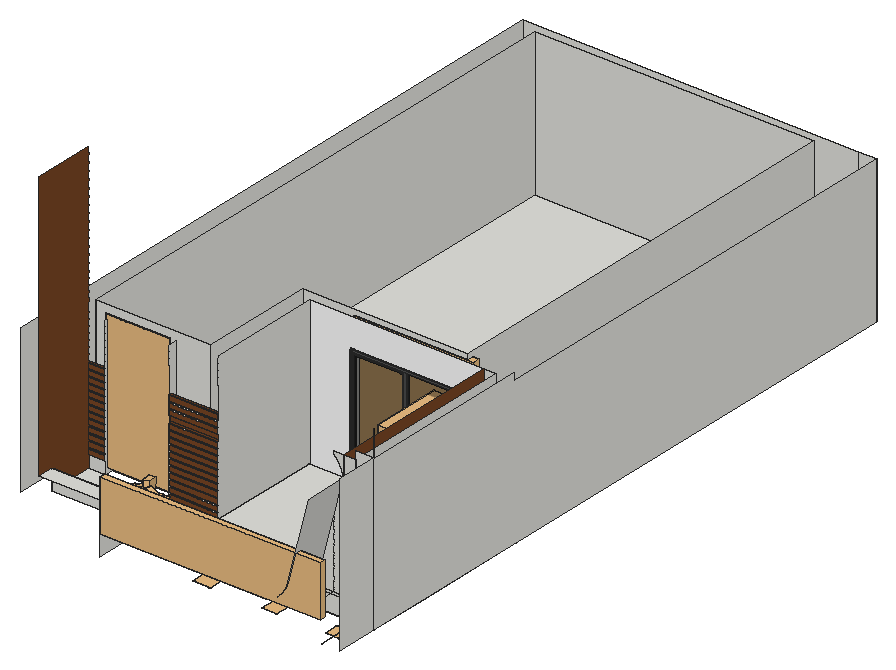
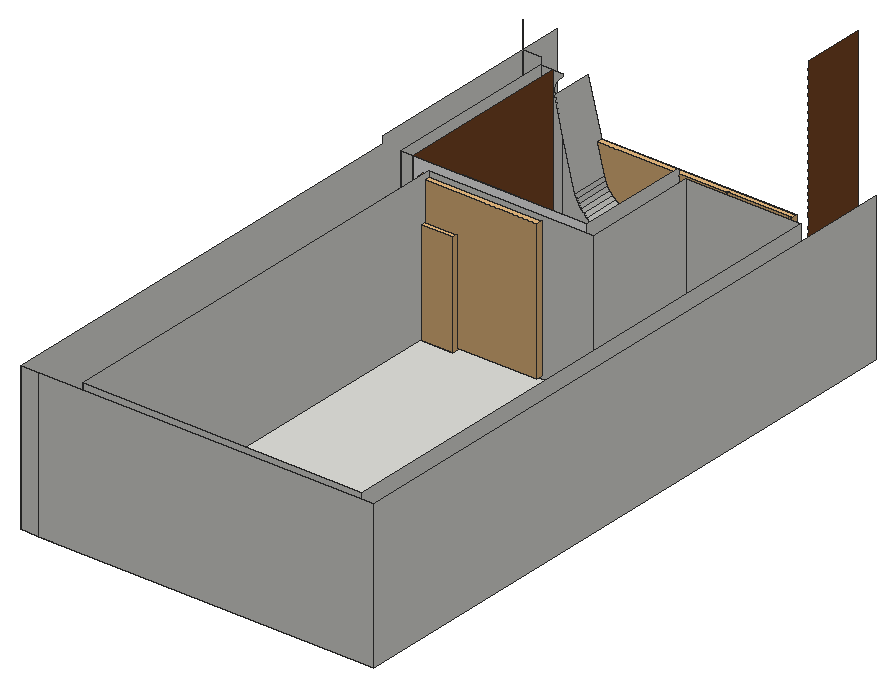
# SketchUp Ruby script. Lengths in inches.
U = 1.inch
M = Sketchup.active_model
def pt(a) = Geom::Point3d.new(a.map { |v| v * U })
def face(e, loops, mat)
  f = e.add_face(loops[0].map { |a| pt(a) })
  loops[1..].each { |l| e.add_face(l.map { |a| pt(a) }).erase! }
  f.material = f.back_material = mat if mat
  f
end
# faces: each face lists its corners as indices into pts; further lists are holes
def faces(e, pts, list, mat = nil) = list.each { |f| face(e, (f[0].is_a?(Array) ? f : [f]).map { |l| l.map { |i| pts[i] } }, mat) }
# xy, xz, yz: faces in a plane at the given z, y or x. An outline is a flat list of corners, or four numbers for a rectangle; further outlines are holes
def ring(l) = l.size == 4 ? [[l[0], l[1]], [l[2], l[1]], [l[2], l[3]], [l[0], l[3]]] : l.each_slice(2).to_a
def flat(e, list, mat, &to3) = list.each { |f| face(e, (f[0].is_a?(Array) ? f : [f]).map { |l| ring(l).map { |u, v| to3.(u, v) } }, mat) }
def xy(e, z, list, mat = nil) = flat(e, list, mat) { |x, y| [x, y, z] }
def xz(e, y, list, mat = nil) = flat(e, list, mat) { |x, z| [x, y, z] }
def yz(e, x, list, mat = nil) = flat(e, list, mat) { |y, z| [x, y, z] }
def lines(e, pts, list) = list.each { |a, b| e.add_line(pt(pts[a]), pt(pts[b])) }
# prism: a flat outline (further loops are holes) pulled along v
def prism(e, loops, v, mat = nil)
  f = face(e, loops, mat); d = Geom::Vector3d.new(v.map { |x| x * U })
  f.pushpull(f.normal.samedirection?(d) ? d.length : -d.length)
end
def box(e, o, s, mat = nil) = prism(e, [[o, [o[0] + s[0], o[1], o[2]], [o[0] + s[0], o[1] + s[1], o[2]], [o[0], o[1] + s[1], o[2]]]], [0, 0, s[2]], mat)
def at(x, y, z, deg = 0) = Geom::Transformation.translation(pt([x, y, z])) * Geom::Transformation.rotation(ORIGIN, Z_AXIS, deg.degrees)
def axes(o, x, y, z) = Geom::Transformation.new([*x, 0, *y, 0, *z, 0, *pt(o).to_a, 1])
def part(name) = M.definitions.add(name)
# library, detail: a bought-in or finely detailed component or shape, given as its bounding box
def library(name, o, s) = part(name).tap { |d| box(d.entities, o, s) }
def detail(e, o, s) = box(e.add_group.entities, o, s)
def put(e, d, t, mat = nil) = e.add_instance(d, t).tap { |i| i.material = mat if mat }
def group(e, t, mat = nil) = e.add_group.tap { |g| g.transformation = t; g.material = mat if mat }.entities
root = M.entities
M.materials.add("Glass_Tinted_Gray").color = [0, 0, 0]
M.materials["Glass_Tinted_Gray"].alpha = 0.125
M.materials.add("Moss 1").color = [97, 97, 43]
M.materials.add("[0135_DarkGray]").color = [81, 81, 81]
M.materials.add("[Color M00]").color = [255, 255, 255]
M.materials.add("[Groundcover_Wood_Mix]").color = [133, 121, 115]
M.materials.add("[Mirror 02]").color = [229, 229, 229]
M.materials.add("[Terrazzo Light Blue]").color = [196, 214, 227]
M.materials.add("[Wood Veneer 01]").color = [120, 70, 37]
c1 = library("Group\#16",[-0.5,-0.5,-0.1],[14.625,14.625,0.2])
c2 = library("Group\#17",[-0.5,-0.5,-0.1],[12,12,0.2])
c3 = library("Group\#18",[-0.5,-0.5,-0.1],[12,12,0.2])
c4 = part("PENTEK_RP Fineline 50S_Sliding_DoorCase_E1")
box(c4.entities,[0,0,0],[1.51,3.66,99.27],"[0135_DarkGray]")
c5 = part("PENTEK_RP Fineline 50S_SlidingDooe_Case_E2")
box(c5.entities,[0,0,0],[96.25,3.66,1.51],"[0135_DarkGray]")
c6 = part("pentek_RP Fineline 50S_SlidingDoor_Case")
put(c6.entities,c4,at(97.76,0,0))
put(c6.entities,c5,at(1.51,0,0))
put(c6.entities,c4,at(0,0,0))
put(c6.entities,c5,at(1.51,0,97.76))
c7 = part("PENTEK_RP Fineline 50S_SlidingDoor_GlazingBead_2")
box(c7.entities,[0,0,0],[0.56,0.59,94.39],"[0135_DarkGray]")
c8 = part("PENTEK_RP Fineline 50S_SlidingDoor_Glass")
box(c8.entities,[0,0,0],[46.58,0.16,94.39],"Glass_Tinted_Gray")
c9 = part("PENTEK_RP Fineline 50S_SlidingDoor_GlazingBead")
box(c9.entities,[0,0,0],[45.47,0.59,0.56],"[0135_DarkGray]")
c10 = part("PENTEK_RP Fineline 50S_SlidingDoor_Leaf_E1")
xy(c10.entities,0,[[0,0,0.93,1.97],[0.93,1.57,1.49,1.97]],"[0135_DarkGray]")
xy(c10.entities,96.25,[[0,0,0.93,0,0.93,1.57,1.49,1.57,1.49,1.97,0,1.97]],"[0135_DarkGray]")
xz(c10.entities,0,[[0,0,0.93,96.25]],"[0135_DarkGray]")
xz(c10.entities,1.57,[[0.93,0,1.49,95.32],[0.93,95.32,1.49,96.25]],"[0135_DarkGray]")
xz(c10.entities,1.97,[[0,0,1.49,96.25]],"[0135_DarkGray]")
yz(c10.entities,0,[[0,0,1.97,96.25]],"[0135_DarkGray]")
yz(c10.entities,0.93,[[0,0,1.57,0.93],[0,0.93,1.57,95.32],[0,95.32,1.57,96.25]],"[0135_DarkGray]")
yz(c10.entities,1.49,[[1.57,0,1.97,95.32],[1.57,95.32,1.97,96.25]],"[0135_DarkGray]")
c11 = part("PENTEK_RP Fineline 50S_SlidingDoor_Leaf_E2")
xy(c11.entities,0,[[0,0,0,1.57,0.56,1.57,0.56,1.97,46.02,1.97,46.02,1.57,46.58,1.57,46.58,0]],"[0135_DarkGray]")
xy(c11.entities,0.93,[[0,0,46.58,1.57]],"[0135_DarkGray]")
xy(c11.entities,1.49,[[0.56,1.57,46.02,1.97]],"[0135_DarkGray]")
xz(c11.entities,0,[[0,0,46.58,0.93]],"[0135_DarkGray]")
xz(c11.entities,1.57,[[0,0,0.56,0.93],[46.02,0,46.58,0.93],[0.56,0.93,46.02,1.49]],"[0135_DarkGray]")
xz(c11.entities,1.97,[[0.56,0,46.02,1.49]],"[0135_DarkGray]")
yz(c11.entities,0,[[0,0,1.57,0.93]],"[0135_DarkGray]")
yz(c11.entities,0.56,[[1.57,0,1.97,0.93],[1.57,0.93,1.97,1.49]],"[0135_DarkGray]")
yz(c11.entities,46.02,[[1.57,0,1.97,0.93],[1.57,0.93,1.97,1.49]],"[0135_DarkGray]")
yz(c11.entities,46.58,[[0,0,1.57,0.93]],"[0135_DarkGray]")
c12 = part("PENTEK_RP Fineline S_SlidingDoor_Leaf1")
put(c12.entities,c7,at(0.93,0,0.93))
put(c12.entities,c7,at(46.96,0,0.93))
put(c12.entities,c8,at(1.49,1.42,0.93))
put(c12.entities,c9,at(1.49,0,0.93))
put(c12.entities,c8,at(1.49,0.59,0.93),"[Terrazzo Light Blue]")
put(c12.entities,c10,at(0,0,0))
put(c12.entities,c10,axes([48.44,0,0],[-1,0,0],[0,1,0],[0,0,1]))
put(c12.entities,c11,axes([0.93,0,96.25],[1,0,0],[0,1,0],[0,0,-1]))
put(c12.entities,c11,at(0.93,0,0))
put(c12.entities,c9,at(1.49,0,94.77))
c13 = part("PENTEK_RP Fineline 50S_SlidingDoor_Leaf2")
put(c13.entities,c8,at(1.49,1.42,0.93))
put(c13.entities,c9,at(1.49,0,94.77))
put(c13.entities,c7,at(46.96,0,0.93))
put(c13.entities,c8,at(1.49,0.59,0.93),"[Mirror 02]")
put(c13.entities,c7,at(0.93,0,0.93))
put(c13.entities,c10,at(0,0,0))
put(c13.entities,c10,axes([48.44,0,0],[-1,0,0],[0,1,0],[0,0,1]))
put(c13.entities,c9,at(1.49,0,0.93))
put(c13.entities,c11,axes([0.93,0,96.25],[1,0,0],[0,1,0],[0,0,-1]))
put(c13.entities,c11,at(0.93,0,0))
c14 = part("PENTEK - Slimmest Steel Sliding Door / Window\#1")
put(c14.entities,c6,at(0,-1.88,-0.09))
put(c14.entities,c12,at(1.51,-2.27,1.42))
put(c14.entities,c13,at(49.32,-0.3,1.42))
c15 = library("plant (1)",[-35.72,-28.42,0],[66.31,67.39,84.38])
c16 = library("panneau+shadow+blanc+bourdon+naturel",[-47.99,-1.29,1.53],[97.82,5.86,114.18])
c17 = library("Decorative screen panel",[0,0,0],[35.43,0.39,70.87])
c18 = part("HCD  9x9 Indo Pot (Square)")
xy(c18.entities,0,[[0,0,9,9]])
xy(c18.entities,0.75,[[0.75,0.75,8.25,8.25]])
xy(c18.entities,7.52,[[0.75,0.75,8.25,8.25]],"Moss 1")
xy(c18.entities,9,[[[0,0,9,9],[0.75,0.75,8.25,8.25]]])
xz(c18.entities,0,[[0,0,9,9]])
xz(c18.entities,0.75,[[0.75,0.75,8.25,7.52],[0.75,7.52,8.25,9]])
xz(c18.entities,8.25,[[0.75,0.75,8.25,7.52],[0.75,7.52,8.25,9]])
xz(c18.entities,9,[[0,0,9,9]])
yz(c18.entities,0,[[0,0,9,9]])
yz(c18.entities,0.75,[[0.75,0.75,8.25,7.52],[0.75,7.52,8.25,9]])
yz(c18.entities,8.25,[[0.75,0.75,8.25,7.52],[0.75,7.52,8.25,9]])
yz(c18.entities,9,[[0,0,9,9]])
c19 = part("Group\#284")
detail(c19.entities,[0,0,0],[2.15,3.79,14.3])
c20 = part("Potted plant")
put(c20.entities,c18,axes([7.375,7.93,0],[1.35,0,0],[0,1.35,0],[0,0,1.35]))
g1 = group(c20.entities,at(34.01,16.59,10.48),"[Groundcover_Wood_Mix]")
put(g1,c19,axes([-21.39,-3.67,0.04],[1.0831,1.67432,0],[1.44561,-0.94233,-0.44822],[0.5095,-0.33212,1.35364]))
put(g1,c19,axes([-19.2,-0.0625,0.04],[0.06577,-1.58752,0],[-1.23,-0.01362,-0.59477],[-0.71488,-0.00792,0.95418]))
put(g1,c19,axes([-20.16,-2.02,1.03],[1.23757,0.97175,0],[0.71987,-0.88743,-0.73204],[0.35645,-0.43942,0.56976]))
put(g1,c19,axes([-20.43,-4.53,0.04],[0.02652,1.58591,0],[1.23087,-0.05659,-0.59477],[0.71539,-0.03289,0.95418]))
put(g1,c19,axes([-19.73,-2.8125,1.03],[-1.55944,0.41251,0],[0.26154,1.08365,-0.73204],[0.12951,0.53658,0.56976]))
put(g1,c19,axes([-19.27,-4.42,0.04],[-1.00701,1.78126,0],[1.48381,0.79245,-0.44822],[0.52297,0.2793,1.35364]))
put(g1,c19,axes([-17.53,-1.6,0.04],[-1.30559,-0.8818,0],[-0.71402,1.01403,-0.59477],[-0.41499,0.58936,0.95418]))
put(g1,c19,axes([-21.8,-1.55,0.04],[2.03404,-0.13573,0],[-0.064,-1.68745,-0.44822],[-0.02256,-0.59474,1.35364]))
put(g1,c19,axes([-19.33,-2.61,1.03],[-1.22683,-0.98484,0],[-0.72899,0.88019,-0.73204],[-0.36097,0.43583,0.56976]))
put(g1,c19,axes([-19.3,-2.11,1.03],[0.27974,-1.57083,0],[-1.11549,-0.16277,-0.73204],[-0.55235,-0.0806,0.56976]))
put(g1,c19,axes([-21.97,-3.02,0.04],[1.31205,0.87256,0],[0.70701,-1.01874,-0.59477],[0.41092,-0.59209,0.95418]))
put(g1,c19,axes([-17.81,-3.69,0.04],[-1.51859,0.55236,0],[0.39363,1.14324,-0.59477],[0.22878,0.66446,0.95418]))
put(g1,c19,axes([-20.2,-2.52,1.03],[-0.299,1.5679,0],[1.11299,0.17632,-0.73204],[0.55111,0.08731,0.56976]))
put(g1,c19,axes([-21.28,-0.49,0.04],[1.33266,-0.92103,0],[-0.68389,-0.99325,-0.59477],[-0.39748,-0.57728,0.95418]))
put(g1,c19,axes([-19.17,-0.27,0.04],[-0.5456,-1.92548,0],[1.93945,-0.59168,-0.26656],[0.28985,-0.08843,1.78359]))
put(g1,c19,axes([-17.96,-1.15,0.04],[-1.27123,-1.53638,0],[-1.33347,1.09526,-0.44822],[-0.46998,0.38602,1.35364]))
put(g1,c19,axes([-19.65,-1.83,1.03],[1.43123,-0.75657,0],[-0.50987,-0.98658,-0.73204],[-0.25247,-0.48851,0.56976]))
put(g1,c19,axes([-16.8,-2.55,0.04],[-1.5632,-0.30402,0],[0.34989,-1.54112,-0.20989],[0.05229,-0.23032,1.4044]))
put(g1,c19,axes([-21.84,-2.79,0.04],[1.97107,0.44464,0],[-0.50241,1.94504,-0.26656],[-0.07509,0.29069,1.78359]))
put(g1,c19,axes([-20.37,0.56,0.04],[0.7463,-1.42646,0],[1.4028,0.68931,-0.20989],[0.20965,0.10302,1.4044]))
put(g1,c19,axes([-17.99,-3.6,0.04],[-1.66024,1.21511,0],[-1.16467,-1.59132,-0.26656],[-0.17406,-0.23783,1.78359]))
put(g1,c19,axes([-21.54,-4.58,0.04],[0.59386,1.45638,0],[-1.47231,0.6251,-0.20989],[-0.22004,0.09342,1.4044]))
put(g1,c19,axes([-19.92,-0.17,0.04],[0.74111,-1.89898,0],[-1.5902,-0.56846,-0.44822],[-0.56047,-0.20035,1.35364]))
c21 = library("Glass Railing",[0,0,0],[139.5,4.76,42])
xy(root,199.25,[[597.67,262.6,597.79,296.73],[416.27,296.73,597.67,296.73,597.67,348.1,597.79,348.1,597.79,440.43,567.52,440.43,567.52,449.58,479.29,449.58,479.29,440.43,445.11,440.43,445.11,348.1,338.58,348.1,338.58,310.29,416.27,310.29],[597.67,296.73,597.79,348.1],[597.79,296.73,612.67,348.1],[612.67,296.73,612.79,442.55],
  [597.79,348.1,612.67,442.55],[338.58,355.13,432.33,355.13,432.33,449.58,567.52,449.58,567.52,804.07,338.58,804.07],[586.74,440.43,597.79,442.55],[586.74,442.55,597.79,811.1],[597.79,442.55,612.67,811.1],
  [612.67,442.55,612.79,811.1]])
xy(root,199.625,[[588.04,296.73,597.42,348.1],[597.42,296.73,597.79,348.1],[588.04,348.1,597.79,440.43]])
xy(root,200.29,[[404.9375,346.73,445.11,348.1]])
xy(root,204.05,[[404.9375,346.73,445.11,348.1]])
xy(root,205.46,[[404.9375,346.73,445.11,348.1]])
xy(root,209.23,[[404.9375,346.73,445.11,348.1]])
xy(root,210.34,[[338.58,346.73,352.5,348.1]])
xy(root,210.64,[[404.9375,346.73,445.11,348.1]])
xy(root,214.06,[[338.58,346.73,352.5,348.1]])
xy(root,214.41,[[404.9375,346.73,445.11,348.1]],"[Wood Veneer 01]")
xy(root,215.78,[[338.58,346.73,352.5,348.1]])
xy(root,215.82,[[404.9375,346.73,445.11,348.1]])
xy(root,215.9375,[[416.0625,262.6,551.49,296.73],[338.58,296.73,416.27,310.29]])
xy(root,219.5,[[338.58,346.73,352.5,348.1]])
xy(root,219.59,[[404.9375,346.73,445.11,348.1]],"[Wood Veneer 01]")
xy(root,221,[[404.9375,346.73,445.11,348.1]])
xy(root,221.21,[[338.58,346.73,352.5,348.1]])
xy(root,224.77,[[404.9375,346.73,445.11,348.1]])
xy(root,224.93,[[338.58,346.73,352.5,348.1]])
xy(root,226.18,[[404.9375,346.73,445.11,348.1]])
xy(root,226.65,[[338.58,346.73,352.5,348.1]])
xy(root,229.95,[[404.9375,346.73,445.11,348.1]])
xy(root,230.37,[[338.58,346.73,352.5,348.1]])
xy(root,231.36,[[404.9375,346.73,445.11,348.1]])
xy(root,232.09,[[338.58,346.73,352.5,348.1]])
xy(root,235.125,[[404.9375,346.73,445.11,348.1]])
xy(root,235.81,[[338.58,346.73,352.5,348.1]])
xy(root,236.54,[[404.9375,346.73,445.11,348.1]])
xy(root,237.22,[[338.58,346.73,352.5,348.1]])
xy(root,240.3,[[404.9375,346.73,445.11,348.1]])
xy(root,240.94,[[338.58,346.73,352.5,348.1]])
xy(root,241.72,[[404.9375,346.73,445.11,348.1]])
xy(root,242.36,[[338.58,346.73,352.5,348.1]])
xy(root,245.48,[[404.9375,346.73,445.11,348.1]])
xy(root,246.08,[[338.58,346.73,352.5,348.1]])
xy(root,246.9,[[404.9375,346.73,445.11,348.1]])
xy(root,247.49,[[338.58,346.73,352.5,348.1]])
xy(root,250.66,[[404.9375,346.73,445.11,348.1]])
xy(root,251.21,[[338.58,346.73,352.5,348.1]])
xy(root,252.08,[[404.9375,346.73,445.11,348.1]])
xy(root,252.62,[[338.58,346.73,352.5,348.1]])
xy(root,255.84,[[404.9375,346.73,445.11,348.1]])
xy(root,256.34,[[338.58,346.73,352.5,348.1]])
xy(root,257.76,[[338.58,346.73,352.5,348.1]])
xy(root,261.48,[[338.58,346.73,352.5,348.1]])
xy(root,262.43,[[404.9375,346.73,445.11,348.1]])
xy(root,262.89,[[338.58,346.73,352.5,348.1]])
xy(root,266.2,[[404.9375,346.73,445.11,348.1]])
xy(root,266.61,[[338.58,346.73,352.5,348.1]])
xy(root,267.61,[[404.9375,346.73,445.11,348.1]])
xy(root,268.02,[[338.58,346.73,352.5,348.1]])
xy(root,271.38,[[404.9375,346.73,445.11,348.1]])
xy(root,271.74,[[338.58,346.73,352.5,348.1]])
xy(root,272.79,[[404.9375,346.73,445.11,348.1]])
xy(root,273.16,[[338.58,346.73,352.5,348.1]])
xy(root,276.56,[[404.9375,346.73,445.11,348.1]])
xy(root,276.875,[[338.58,346.73,352.5,348.1]])
xz(root,296.73,[[416.27,199.25,597.67,199.625],[597.67,199.25,597.79,199.625],[597.79,199.25,612.67,325.25],[612.67,199.25,612.79,346.9375],[416.27,199.625,588.04,213.375],
  [588.04,199.625,597.79,213.375],[416.27,213.375,588.04,215.9375],[588.04,213.375,597.79,215.9375],[551.49,215.9375,554.51,216.95,557.62,218.48,560.5,220.41,563.11,222.7,565.38,225.32,567.3,228.21,568.81,231.33,569.9,234.625,579.8,272.97,579.8,215.9375],[579.8,215.9375,579.8,272.97,587.03,300.95,587.16,304.37,586.56,307.74,585.26,310.9,583.31,313.72,580.81,316.05,579.8,316.65,579.8,319.25,588.04,319.25,588.04,215.9375],
  [588.04,215.9375,597.79,319.25]])
xz(root,310.29,[[338.58,199.25,416.27,215.9375]])
xz(root,346.73,[[404.9375,200.29,445.11,204.05],[404.9375,205.46,445.11,209.23],[338.58,210.34,352.5,214.06],[404.9375,210.64,445.11,214.41],[338.58,215.78,352.5,219.5],
  [404.9375,215.82,445.11,219.59],[404.9375,221,445.11,224.77],[338.58,221.21,352.5,224.93],[404.9375,226.18,445.11,229.95],[338.58,226.65,352.5,230.37],
  [404.9375,231.36,445.11,235.125],[338.58,232.09,352.5,235.81],[404.9375,236.54,445.11,240.3],[338.58,237.22,352.5,240.94],[404.9375,241.72,445.11,245.48],
  [338.58,242.36,352.5,246.08],[404.9375,246.9,445.11,250.66],[338.58,247.49,352.5,251.21],[404.9375,252.08,445.11,255.84],[338.58,252.62,352.5,256.34],
  [338.58,257.76,352.5,261.48],[404.9375,262.43,445.11,266.2],[338.58,262.89,352.5,266.61],[404.9375,267.61,445.11,271.38],[338.58,268.02,352.5,271.74],
  [404.9375,272.79,445.11,276.56],[338.58,273.16,352.5,276.875]],"[Wood Veneer 01]")
xz(root,348.1,[[338.58,199.25,352.5,210.34],[404.9375,199.25,445.11,200.29],[597.67,199.25,597.79,199.625],[404.9375,272.79,445.11,276.56]])
xz(root,348.1,[[404.9375,204.05,445.11,205.46],[404.9375,209.23,445.11,210.64],[338.58,214.06,352.5,215.78],[404.9375,214.41,445.11,215.82],[338.58,219.5,352.5,221.21],
  [404.9375,219.59,445.11,221],[404.9375,224.77,445.11,226.18],[338.58,224.93,352.5,226.65],[404.9375,229.95,445.11,231.36],[338.58,230.37,352.5,232.09],
  [404.9375,235.125,445.11,236.54],[338.58,235.81,352.5,237.22],[404.9375,240.3,445.11,241.72],[338.58,240.94,352.5,242.36],[404.9375,245.48,445.11,246.9],
  [338.58,246.08,352.5,247.49],[404.9375,250.66,445.11,252.08],[338.58,251.21,352.5,252.62],[404.9375,255.84,445.11,257.25],[338.58,256.34,352.5,257.76],
  [404.9375,257.25,445.11,261.02],[404.9375,261.02,445.11,262.43],[338.58,261.48,352.5,262.89],[404.9375,266.2,445.11,267.61],[338.58,266.61,352.5,268.02],
  [404.9375,271.38,445.11,272.79],[338.58,271.74,352.5,273.16],[404.9375,276.56,445.11,277.97],[338.58,276.875,352.5,278.29]],"[Wood Veneer 01]")
xz(root,355.13,[[338.58,199.25,432.33,319.25]])
xz(root,440.43,[[445.11,199.25,479.29,199.625],[567.52,199.25,586.74,199.625],[586.74,199.25,597.79,199.625],[588.04,199.625,597.79,319.25]])
xz(root,440.43,[[445.11,199.625,479.29,199.625,479.29,296,567.52,296,567.52,199.625,588.04,199.625,588.04,319.25,445.11,319.25]],"[Color M00]")
xz(root,449.58,[[432.33,199.25,432.33,319.25,567.52,319.25,567.52,296,479.29,296,479.29,199.25],[479.29,199.25,567.52,199.625]])
xz(root,804.07,[[338.58,199.25,567.52,319.25]])
xz(root,811.1,[[323.43,199.25,597.79,319.25],[597.79,199.25,612.79,319.25]])
yz(root,323.43,[[296.73,199.25,811.1,319.25]])
yz(root,338.58,[[355.13,199.25,804.07,319.25]])
yz(root,338.58,[[310.29,199.25,348.1,199.25,348.1,210.34,346.73,210.34,346.73,214.06,348.1,214.06,348.1,215.78,346.73,215.78,346.73,219.5,348.1,219.5,348.1,221.21,346.73,221.21,346.73,224.93,348.1,224.93,348.1,226.65,346.73,226.65,346.73,230.37,348.1,230.37,348.1,232.09,346.73,232.09,346.73,235.81,348.1,235.81,348.1,237.22,346.73,237.22,346.73,240.94,348.1,240.94,348.1,242.36,346.73,242.36,346.73,246.08,348.1,246.08,348.1,247.49,346.73,247.49,346.73,251.21,348.1,251.21,348.1,252.62,346.73,252.62,346.73,256.34,348.1,256.34,348.1,257.76,346.73,257.76,346.73,261.48,348.1,261.48,348.1,262.89,346.73,262.89,346.73,266.61,348.1,266.61,348.1,268.02,346.73,268.02,346.73,271.74,348.1,271.74,348.1,273.16,346.73,273.16,346.73,276.875,348.1,276.875,348.1,278.29,346.73,278.29,346.73,282.01,348.1,282.01,348.1,283.42,346.73,283.42,346.73,287.14,348.1,287.14,348.1,288.56,346.73,288.56,346.73,292.28,348.1,292.28,348.1,293.6875,346.73,293.6875,346.73,297.41,348.1,297.41,348.1,298.82,346.73,298.82,346.73,302.54,348.1,302.54,348.1,303.96,346.73,303.96,346.73,307.68,348.1,307.68,348.1,309.09,346.73,309.09,346.73,312.81,348.1,312.81,348.1,314.22,346.73,314.22,346.73,321.49,348.1,321.49,348.1,324.09,346.73,324.09,346.73,327.93,348.1,327.93,348.1,329.07,346.73,329.07,346.73,332.9,348.1,332.9,348.1,334.04,346.73,334.04,346.73,337.875,348.1,337.875,348.1,339.02,346.73,339.02,346.73,342.85,348.1,342.85,348.1,343.99,346.73,343.99,346.73,349.02,348.1,349.02,348.1,350.07,346.73,350.07,346.73,355.09,348.1,355.09,348.1,356.14,346.73,356.14,346.73,361.17,348.1,361.17,348.1,362.21,346.73,362.21,346.73,367.24,348.1,367.24,348.1,368.29,346.73,368.29,346.73,373.32,348.1,373.32,348.1,374.36,346.73,374.36,346.73,379.39,348.1,379.39,348.1,380.4375,346.73,380.4375,346.73,385.46,348.1,385.46,348.1,386.51,346.73,386.51,346.73,391.54,348.1,391.54,348.1,392.59,346.73,392.59,346.73,397.61,348.1,397.61,348.1,398.66,346.73,398.66,346.73,403.6875,348.1,403.6875,348.1,404.97,346.73,404.97,346.73,410,348.1,410,348.1,411.28,346.73,411.28,346.73,416.3125,348.1,416.3125,348.1,417.6,346.73,417.6,346.73,422.625,348.1,422.625,348.1,423.91,346.73,423.91,346.73,428.9375,348.1,428.9375,348.1,430.22,346.73,430.22,346.73,435.25,296.73,435.25,296.73,215.9375,310.29,215.9375]],"[Wood Veneer 01]")
yz(root,352.5,[[348.1,199.25,354.42,199.25,354.42,312.81,346.73,312.81,346.73,309.09,348.1,309.09,348.1,307.68,346.73,307.68,346.73,303.96,348.1,303.96,348.1,302.54,346.73,302.54,346.73,298.82,348.1,298.82,348.1,297.41,346.73,297.41,346.73,293.6875,348.1,293.6875,348.1,292.28,346.73,292.28,346.73,288.56,348.1,288.56,348.1,287.14,346.73,287.14,346.73,283.42,348.1,283.42,348.1,282.01,346.73,282.01,346.73,278.29,348.1,278.29,348.1,276.875,346.73,276.875,346.73,273.16,348.1,273.16,348.1,271.74,346.73,271.74,346.73,268.02,348.1,268.02,348.1,266.61,346.73,266.61,346.73,262.89,348.1,262.89,348.1,261.48,346.73,261.48,346.73,257.76,348.1,257.76,348.1,256.34,346.73,256.34,346.73,252.62,348.1,252.62,348.1,251.21,346.73,251.21,346.73,247.49,348.1,247.49,348.1,246.08,346.73,246.08,346.73,242.36,348.1,242.36,348.1,240.94,346.73,240.94,346.73,237.22,348.1,237.22,348.1,235.81,346.73,235.81,346.73,232.09,348.1,232.09,348.1,230.37,346.73,230.37,346.73,226.65,348.1,226.65,348.1,224.93,346.73,224.93,346.73,221.21,348.1,221.21,348.1,219.5,346.73,219.5,346.73,215.78,348.1,215.78,348.1,214.06,346.73,214.06,346.73,210.34,348.1,210.34]])
yz(root,404.9375,[[348.1,199.25,348.1,200.29,346.73,200.29,346.73,204.05,348.1,204.05,348.1,205.46,346.73,205.46,346.73,209.23,348.1,209.23,348.1,210.64,346.73,210.64,346.73,214.41,348.1,214.41,348.1,215.82,346.73,215.82,346.73,219.59,348.1,219.59,348.1,221,346.73,221,346.73,224.77,348.1,224.77,348.1,226.18,346.73,226.18,346.73,229.95,348.1,229.95,348.1,231.36,346.73,231.36,346.73,235.125,348.1,235.125,348.1,236.54,346.73,236.54,346.73,240.3,348.1,240.3,348.1,241.72,346.73,241.72,346.73,245.48,348.1,245.48,348.1,246.9,346.73,246.9,346.73,250.66,348.1,250.66,348.1,252.08,346.73,252.08,346.73,255.84,348.1,255.84,348.1,262.43,346.73,262.43,346.73,266.2,348.1,266.2,348.1,267.61,346.73,267.61,346.73,271.38,348.1,271.38,348.1,298.69,346.73,298.69,346.73,302.45,348.1,302.45,348.1,303.86,346.73,303.86,346.73,307.63,348.1,307.63,348.1,309.04,346.73,309.04,346.73,312.81,354.42,312.81,354.42,199.25],[346.73,272.79,348.1,276.56]])
yz(root,416.0625,[[262.6,199.25,296.73,215.9375]])
yz(root,416.27,[[296.73,199.25,310.29,215.9375]])
yz(root,432.33,[[355.13,199.25,449.58,319.25]])
yz(root,445.11,[[348.1,199.25,440.43,199.625],[348.1,199.625,440.43,199.625,440.43,319.25,348.1,319.25,348.1,317.66,346.73,317.66,346.73,314.22,348.1,314.22,348.1,312.81,346.73,312.81,346.73,309.04,348.1,309.04,348.1,307.63,346.73,307.63,346.73,303.86,348.1,303.86,348.1,302.45,346.73,302.45,346.73,298.69,348.1,298.69,348.1,271.38,346.73,271.38,346.73,267.61,348.1,267.61,348.1,266.2,346.73,266.2,346.73,262.43,348.1,262.43,348.1,255.84,346.73,255.84,346.73,252.08,348.1,252.08,348.1,250.66,346.73,250.66,346.73,246.9,348.1,246.9,348.1,245.48,346.73,245.48,346.73,241.72,348.1,241.72,348.1,240.3,346.73,240.3,346.73,236.54,348.1,236.54,348.1,235.125,346.73,235.125,346.73,231.36,348.1,231.36,348.1,229.95,346.73,229.95,346.73,226.18,348.1,226.18,348.1,224.77,346.73,224.77,346.73,221,348.1,221,348.1,219.59,346.73,219.59,346.73,215.82,348.1,215.82,348.1,214.41,346.73,214.41,346.73,210.64,348.1,210.64,348.1,209.23,346.73,209.23,346.73,205.46,348.1,205.46,348.1,204.05,346.73,204.05,346.73,200.29,348.1,200.29],[346.73,272.79,348.1,276.56]])
yz(root,479.29,[[440.43,199.25,449.58,199.625],[440.43,199.625,449.58,296]])
yz(root,567.52,[[440.43,199.25,449.58,199.625],[449.58,199.25,804.07,319.25],[440.43,199.625,449.58,296]])
yz(root,588.04,[[296.73,199.625,440.43,319.25]],"[Wood Veneer 01]")
yz(root,597.79,[[348.1,199.25,440.43,199.625],[296.73,199.625,440.43,319.25]])
yz(root,612.67,[[262.6,199.25,296.73,325.25]])
yz(root,612.79,[[296.73,199.25,811.1,199.25,811.1,319.25,440.43,319.25,440.43,325.25,296.73,325.25]])
p = [[551.49,262.6,215.9375],[554.51,262.6,216.95],[554.51,296.73,216.95],[551.49,296.73,215.9375],[557.62,262.6,218.48],[557.62,296.73,218.48],
  [560.5,262.6,220.41],[560.5,296.73,220.41],[563.11,262.6,222.7],[563.11,296.73,222.7],[565.38,262.6,225.32],[565.38,296.73,225.32],
  [567.3,262.6,228.21],[567.3,296.73,228.21],[568.81,262.6,231.33],[568.81,296.73,231.33],[569.9,262.6,234.625],[569.9,296.73,234.625],
  [587.03,296.73,300.95],[579.8,296.73,272.97],[587.03,262.6,300.95],[579.8,262.6,215.9375],[579.8,296.73,215.9375]]
faces(root,p,[[0,1,2,3],[1,4,5,2],[4,6,7,5],[6,8,9,7],[8,10,11,9],[10,12,13,11],[12,14,15,13],[14,16,17,15],
  [18,19,17,16,20]])
lines(root,p,[[21,22]])
put(root,c1,at(470.25,290.64,188.0625))
put(root,c2,at(527.27,290.71,188.0625))
put(root,c3,at(578.89,290.71,188.0625))
put(root,c14,axes([480.1,440.43,197.17],[0.89,0,0],[0,1,0],[0,0,1]))
put(root,c15,at(576.77,419.32,199.25))
put(root,c16,at(523.4,449.58,199.25))
put(root,c17,axes([351.6875,348.59,204.68],[1.4799,0,0],[0,1.58558,0],[0,0,1.58558]),"[Color M00]")
put(root,c20,axes([415.43,269.4,204.9],[1.19,0,0],[0,1.19,0],[0,0,1.19]))
put(root,c21,axes([416.0625,262.6,215.9375],[1.29451,0,0],[0,1,0],[0,0,1]))
